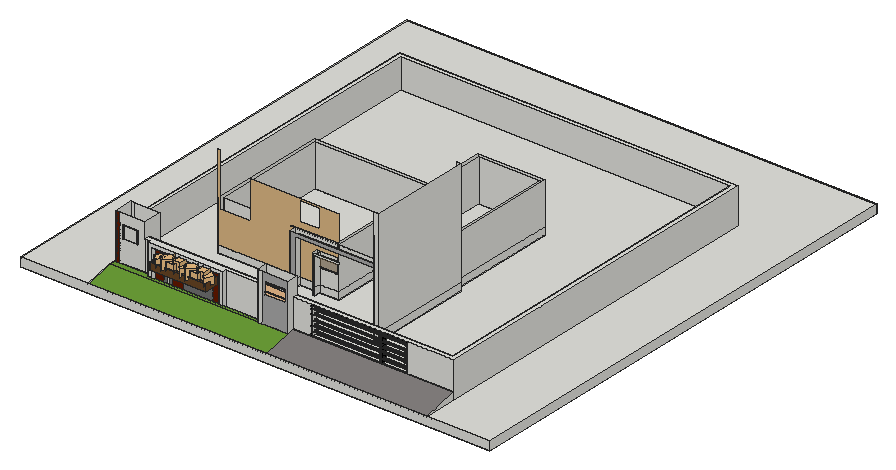
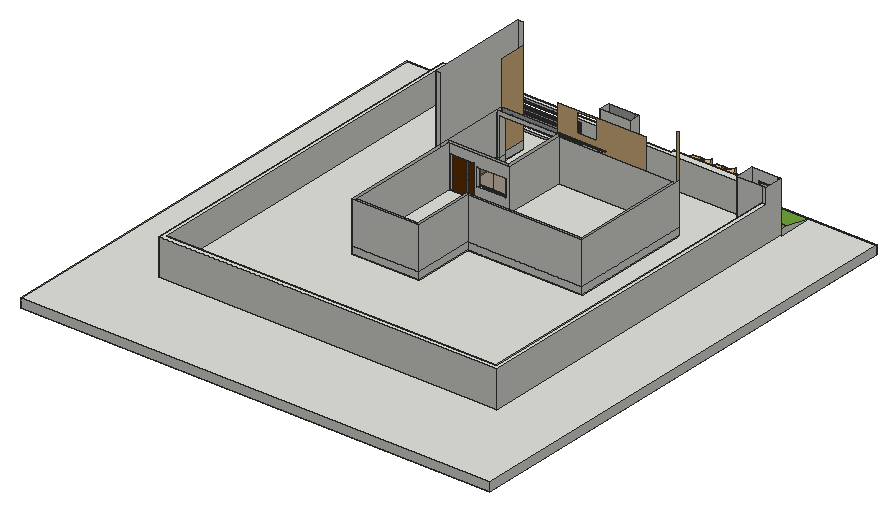
# SketchUp Ruby script. Lengths in millimetres.
U = 1.mm
M = Sketchup.active_model
def pt(a) = Geom::Point3d.new(a.map { |v| v * U })
def face(e, loops, mat)
  f = e.add_face(loops[0].map { |a| pt(a) })
  loops[1..].each { |l| e.add_face(l.map { |a| pt(a) }).erase! }
  f.material = f.back_material = mat if mat
  f
end
# faces: each face lists its corners as indices into pts; further lists are holes
def faces(e, pts, list, mat = nil) = list.each { |f| face(e, (f[0].is_a?(Array) ? f : [f]).map { |l| l.map { |i| pts[i] } }, mat) }
# xy, xz, yz: faces in a plane at the given z, y or x. An outline is a flat list of corners, or four numbers for a rectangle; further outlines are holes
def ring(l) = l.size == 4 ? [[l[0], l[1]], [l[2], l[1]], [l[2], l[3]], [l[0], l[3]]] : l.each_slice(2).to_a
def flat(e, list, mat, &to3) = list.each { |f| face(e, (f[0].is_a?(Array) ? f : [f]).map { |l| ring(l).map { |u, v| to3.(u, v) } }, mat) }
def xy(e, z, list, mat = nil) = flat(e, list, mat) { |x, y| [x, y, z] }
def xz(e, y, list, mat = nil) = flat(e, list, mat) { |x, z| [x, y, z] }
def yz(e, x, list, mat = nil) = flat(e, list, mat) { |y, z| [x, y, z] }
def lines(e, pts, list) = list.each { |a, b| e.add_line(pt(pts[a]), pt(pts[b])) }
# prism: a flat outline (further loops are holes) pulled along v
def prism(e, loops, v, mat = nil)
  f = face(e, loops, mat); d = Geom::Vector3d.new(v.map { |x| x * U })
  f.pushpull(f.normal.samedirection?(d) ? d.length : -d.length)
end
def box(e, o, s, mat = nil) = prism(e, [[o, [o[0] + s[0], o[1], o[2]], [o[0] + s[0], o[1] + s[1], o[2]], [o[0], o[1] + s[1], o[2]]]], [0, 0, s[2]], mat)
def at(x, y, z, deg = 0) = Geom::Transformation.translation(pt([x, y, z])) * Geom::Transformation.rotation(ORIGIN, Z_AXIS, deg.degrees)
def axes(o, x, y, z) = Geom::Transformation.new([*x, 0, *y, 0, *z, 0, *pt(o).to_a, 1])
def part(name) = M.definitions.add(name)
# library, detail: a bought-in or finely detailed component or shape, given as its bounding box
def library(name, o, s) = part(name).tap { |d| box(d.entities, o, s) }
def detail(e, o, s) = box(e.add_group.entities, o, s)
def put(e, d, t, mat = nil) = e.add_instance(d, t).tap { |i| i.material = mat if mat }
def group(e, t, mat = nil) = e.add_group.tap { |g| g.transformation = t; g.material = mat if mat }.entities
root = M.entities
M.materials.add("Material__1").color = [95, 70, 46]
M.materials.add("[Color B08]").color = [102, 25, 0]
M.materials.add("[Color C02]").color = [255, 204, 153]
M.materials.add("[Color C06]").color = [204, 102, 0]
M.materials.add("[Color C08]").color = [102, 51, 0]
M.materials.add("[Color M03]").color = [170, 170, 170]
M.materials.add("[Color M05]").color = [114, 114, 114]
M.materials.add("[Color M09]").color = [0, 0, 0]
M.materials.add("[Fencing Wood Old]").color = [132, 128, 126]
M.materials.add("[Grass Dark Green]").color = [106, 157, 55]
M.materials.add("[Translucent Glass Gray]").color = [128, 100, 65]
M.materials["[Translucent Glass Gray]"].alpha = 0.5
M.materials.add("[Wallpaper Stripe]1").color = [222, 185, 133]
M.materials.add("[Wood Veneer 01]").color = [104, 70, 37]
c1 = library("Areca palm plant",[0,0,0],[1247.1,929.7,1383.3])
c2 = library("Group20\#1",[-528.7,-433.9,96.3],[1012.6,1001.6,952.6])
c3 = library("Group\#130",[-186.5,-30.4,0],[982.4,909.6,1245.7])
c4 = library("Group38\#2",[355.8,722.5,-595.2],[471.9,465.1,987.8])
c5 = library("Group\#18",[-2151.2,-2287.7,-9.3],[4483.3,4448.3,4353.7])
c6 = library("Group\#74",[-2151.2,-2287.7,-9.3],[4483.3,4448.3,4353.7])
c7 = library("Group20\#2",[-528.7,-433.9,96.3],[1012.6,1001.6,952.6])
xy(root,-1719.3,[[[0,0,37484,38608],[24317.2,4921.6,24679,4921.6,24679,13178.8,24317.2,13178.8,24317.2,21945.9,18983.2,21945.9,18983.2,17069.1,9839.2,17069.1,9839.2,7467.9,15925.7,7467.9,15925.7,7006,16385.5,7006,16385.5,7467.9,17737,7467.9,17737,7006,17916.4,7006,17916.4,7467.9,19440.4,7467.9,19440.4,12344.7,24317.2,12344.7,24317.2,7467.9,24068.1,7467.9,24068.1,7006,24317.2,7006]]])
xy(root,-1062,[[0,0,5401.7,0,5401.7,2705.1,5428.7,2705.1,5428.7,31078.5,32435.2,31078.5,32435.2,0,37484,0,37484,38608,0,38608],[5401.7,0,32435.2,0,32435.2,2705.1,18869,2705.1,18869,2189.2,17189.8,2189.2,17189.8,2457.5,8186.8,2457.5,8186.8,2705.1,5401.7,2705.1],[8573.9,2457.5,13875.2,2705.1],[14222.2,2457.5,17189.8,2705.1]])
xy(root,-597.6,[[5401.7,2189.2,17189.8,2189.2,17189.8,2457.5,8186.8,2457.5,8186.8,2705.1,5401.7,2705.1]],"[Grass Dark Green]")
xy(root,-582.6,[[[7761.5,3056,32084.3,3056,32084.3,30727.6,5779.6,30727.6,5779.6,4232.4,7761.5,4232.4],[24317.2,4921.6,24317.2,7006,24068.1,7006,24068.1,7467.9,24317.2,7467.9,24317.2,12344.7,19440.4,12344.7,19440.4,7467.9,17916.4,7467.9,17916.4,7006,17737,7006,17737,7467.9,16385.5,7467.9,16385.5,7006,15925.7,7006,15925.7,7467.9,9839.2,7467.9,9839.2,17069.1,18983.2,17069.1,18983.2,21945.9,24317.2,21945.9,24317.2,13178.8,24679,13178.8,24679,4921.6]]])
xy(root,-453.1,[[21185.9,2705.1,26553.4,3056],[26740.8,2705.1,28682.4,3056]])
xy(root,-60,[[26604.3,2675,26678.9,2705.1]])
xy(root,0,[[24317.2,4921.6,24679,13178.8],[15925.7,7006,16385.5,7006,16385.5,7467.9,19440.4,7467.9,19440.4,12344.7,22064.1,12344.7,22064.1,12573.3,19211.8,12573.3,19211.8,7696.5,10067.8,7696.5,10067.8,16840.5,19211.8,16840.5,19211.8,21717.3,24088.6,21717.3,24088.6,12573.3,23941.7,12573.3,23941.7,12344.7,24317.2,12344.7,24317.2,21945.9,18983.2,21945.9,18983.2,17069.1,9839.2,17069.1,9839.2,7467.9,15925.7,7467.9],[17737,7006,17916.4,7467.9],[24068.1,7006,24317.2,7467.9],[10067.8,7696.5,19211.8,7696.5,19211.8,12573.3,24088.6,12573.3,24088.6,21717.3,19211.8,21717.3,19211.8,16840.5,10067.8,16840.5],
  [22064.1,12344.7,22164,12344.7,22164,12522.5,23841.8,12522.5,23841.8,12344.7,23941.7,12344.7,23941.7,12573.3,22064.1,12573.3],[22164,12344.7,23841.8,12522.5]])
xy(root,143.2,[[26604.3,2675,26678.9,2705.1]])
xy(root,489.4,[[9066,1643.1,13519,2705.1]])
xy(root,651.3,[[9192.3,1769.3,13392.7,2705.1]])
xy(root,971.6,[[19543.5,12344.7,21847.6,12573.3]])
xy(root,1081.4,[[23379.6,12446.3,23760.6,12522.5]])
xy(root,1091,[[9066,1643.1,13519,1643.1,13519,2705.1,13392.7,2705.1,13392.7,1769.3,9192.3,1769.3,9192.3,2705.1,9066,2705.1]],"[Wood Veneer 01]")
xy(root,1157.6,[[23379.6,12446.3,23760.6,12522.5]])
xy(root,1161.7,[[6020.4,2705.1,7206.3,2730.5]])
xy(root,1237.5,[[6096.2,2705.1,7130.5,2730.5]])
xy(root,1413.2,[[26604.3,2675,26678.9,2705.1]])
xy(root,1565.9,[[8573.9,2457.5,13875.2,2705.1]])
xy(root,1610.1,[[26604.3,2675,26678.9,2705.1]],"[Color M03]")
xy(root,1691.4,[[21185.9,2705.1,26553.4,3056],[26740.8,2705.1,28682.4,3056]])
xy(root,1820.9,[[8186.8,2457.5,14222.2,2457.5,14222.2,2705.1,17189.8,2705.1,17189.8,3052.8,19635.7,3052.8,19635.7,2705.1,32435.2,2705.1,32435.2,31078.5,5428.7,31078.5,5428.7,4232.4,5779.6,4232.4,5779.6,30727.6,32084.3,30727.6,32084.3,3056,7761.5,3056,7761.5,2705.1,8186.8,2705.1]])
xz(root,0,[[0,-1719.3,37484,-1062]])
xz(root,1643.1,[[9066,489.4,13519,1091]],"[Wood Veneer 01]")
xz(root,1769.3,[[9192.3,651.3,13392.7,1091]])
xz(root,2189.2,[[17189.8,-1062,17330.6,-597.6],[17330.6,-1062,17575.1,-597.6],[17575.1,-1062,18869,-597.6],[17330.6,-597.6,17575.1,3141.7]])
xz(root,2189.2,[[17767.7,1526.9,19436.2,1764.4],[17767.7,1764.4,19436.2,1796.7],[17767.7,1796.7,19436.2,2287.5]],"[Color C02]")
xz(root,2189.2,[[17189.8,-597.6,17330.6,3141.7],[[17575.1,-597.6,19635.7,3141.7],[17767.7,1526.9,19436.2,2536.5]]],"[Color M03]")
xz(root,2457.5,[[8186.8,-1062,8573.9,-597.6],[8573.9,-1062,13875.2,-597.6],[13875.2,-1062,14222.2,-597.6],[14222.2,-1062,17189.8,-597.6],[8186.8,-597.6,8573.9,-597.6,8573.9,1565.9,13875.2,1565.9,13875.2,-597.6,14222.2,-597.6,14222.2,1820.9,8186.8,1820.9]])
xz(root,2675,[[26604.3,-60,26678.9,143.2],[26604.3,1413.2,26678.9,1610.1]],"[Color M03]")
xz(root,2705.1,[[5401.7,-1062,5428.7,-597.6],[5428.7,-1062,5561.2,-597.6],[5561.2,-1062,5760.5,-597.6],[5760.5,-1062,7761.5,-597.6],[7761.5,-1062,8186.8,-597.6],
  [9523.8,-1062,9761.8,489.4],[14222.2,-1062,17189.8,1820.9],[18869,-1062,21056.4,-488.2],[21056.4,-1062,28811.9,-488.2],[28811.9,-1062,32435.2,-488.2],
  [5428.7,-597.6,5561.2,2994],[[5760.5,-597.6,7761.5,2994],[6020.4,1161.7,7206.3,2222.2]],[7761.5,-597.6,8186.8,1820.9],[19635.7,-488.2,21056.4,1820.9],[28811.9,-488.2,32435.2,1820.9],
  [26604.3,-60,26678.9,143.2],[9523.8,651.3,9761.8,1565.9],[6096.2,1237.5,7130.5,2146.4]])
xz(root,2705.1,[[8573.9,-1062,9295.9,-1062,9295.9,489.4,9066,489.4,9066,1091,9192.3,1091,9192.3,651.3,9295.9,651.3,9295.9,1565.9,8573.9,1565.9],[9989.6,-1062,10808,489.4],[13214.2,-1062,13875.2,-1062,13875.2,1565.9,13214.2,1565.9,13214.2,651.3,13392.7,651.3,13392.7,1091,13519,1091,13519,489.4,13214.2,489.4],[5561.2,-597.6,5760.5,2994],[9989.6,651.3,10808,1565.9]],"[Color B08]")
xz(root,2705.1,[[9295.9,-1062,9523.8,489.4],[9761.8,-1062,9989.6,489.4],[10808,-1062,13214.2,489.4],[9295.9,651.3,9523.8,1565.9],[9761.8,651.3,9989.6,1565.9],
  [10808,651.3,13214.2,1565.9]],"[Color M05]")
xz(root,2705.1,[[[21056.4,-488.2,28811.9,1820.9],[21185.9,-453.1,28682.4,1691.4]],[[26553.4,-453.1,26740.8,1691.4],[26604.3,-60,26678.9,143.2],[26604.3,1413.2,26678.9,1610.1]]],"[Color M09]")
xz(root,2730.5,[[[6020.4,1161.7,7206.3,2222.2],[6096.2,1237.5,7130.5,2146.4]]])
xz(root,3052.8,[[17189.8,1820.9,19635.7,3141.7]])
xz(root,3056,[[[7761.5,-582.6,32084.3,1820.9],[21185.9,-453.1,26553.4,1691.4],[26740.8,-453.1,28682.4,1691.4]]])
xz(root,4232.4,[[5779.6,-582.6,7761.5,2994],[5428.7,1820.9,5779.6,2994]])
xz(root,4921.6,[[24317.2,-1719.3,24679,-582.6],[24317.2,-582.6,24679,0],[24317.2,0,24679,8532.8]])
xz(root,7006,[[15925.7,-1719.3,16385.5,-582.6],[17737,-1719.3,17916.4,-582.6],[24068.1,-1719.3,24317.2,-582.6],[15925.7,-582.6,16385.5,0],[17737,-582.6,17916.4,0],
  [24068.1,-582.6,24317.2,0],[17737,0,17916.4,0,17916.4,2265.6,19853.2,2265.6,19853.2,2420.1,17737,2420.1]])
xz(root,7006,[[15925.7,0,16385.5,0,16385.5,3053.2,24068.1,3053.2,24068.1,0,24317.2,0,24317.2,3352.8,15925.7,3352.8]],"[Color M03]")
xz(root,7467.9,[[9839.2,-1719.3,15925.7,-582.6],[16385.5,-1719.3,17737,-582.6],[17916.4,-1719.3,19440.4,-582.6],[24068.1,-1719.3,24317.2,-582.6],[9839.2,-582.6,15925.7,0],
  [16385.5,-582.6,17737,0],[17916.4,-582.6,19440.4,0],[24068.1,-582.6,24317.2,0],[17737,0,17916.4,2265.6],[17916.4,0,19440.4,1219.2],
  [24068.1,0,24068.1,3053.2,19440.4,3053.2,19440.4,3352.8,24317.2,3352.8,24317.2,0]])
xz(root,7467.9,[[[17916.4,1219.2,19440.4,2133.6],[17964.1,1266.9,19392.7,2085.9]]],"[Color B08]")
xz(root,7467.9,[[17964.1,1266.9,19392.7,2085.9]],"[Translucent Glass Gray]")
xz(root,7467.9,[[[9839.2,0,15925.7,0,15925.7,3352.8,23273.7,3352.8,23273.7,3388.1,15532.7,3388.1,15532.7,3920.5,15634.5,3920.5,15634.5,3497.3,19430.1,3497.3,19430.1,5591.3,12413.6,5591.3,12413.6,2590.3,9937.1,2590.3,9937.1,6850.1,9839.2,6850.1],[16385.5,3962.4,17916.4,5486.4]],[16385.5,0,17737,0,17737,2420.1,19440.4,2420.1,19440.4,3053.2,16385.5,3053.2]],"[Wallpaper Stripe]1")
xz(root,7696.5,[[10067.8,0,19211.8,3352.8]])
xz(root,12344.7,[[19440.4,-1719.3,24317.2,-582.6],[19440.4,-582.6,24317.2,0],[[19440.4,0,22064.1,0,22064.1,2627.4,23941.7,2627.4,23941.7,0,24317.2,0,24317.2,3352.8,19440.4,3352.8],[19543.5,971.6,21847.6,2395.6]]])
xz(root,12344.7,[[22064.1,0,22164,0,22164,2527.5,23841.8,2527.5,23841.8,0,23941.7,0,23941.7,2627.4,22064.1,2627.4]],"[Color C08]")
xz(root,12344.7,[[[19543.5,971.6,21847.6,2395.6],[19613.2,1041.2,21777.9,2325.9]]],"[Color M09]")
xz(root,12344.7,[[19613.2,1041.2,20695.5,2325.9],[20695.5,1041.2,21777.9,2325.9]],"[Translucent Glass Gray]")
xz(root,12446.3,[[23379.6,1081.4,23760.6,1157.6]])
xz(root,12522.5,[[22528.5,0,22698.2,2527.5]],"[Color C06]")
xz(root,12522.5,[[22164,0,22528.5,2527.5],[[22698.2,0,23841.8,2527.5],[23379.6,1081.4,23760.6,1157.6]]],"[Color C08]")
xz(root,12573.3,[[[19211.8,0,19211.8,3352.8,24088.6,3352.8,24088.6,0,23941.7,0,23941.7,2627.4,22064.1,2627.4,22064.1,0],[19543.5,971.6,21847.6,2395.6]]])
xz(root,13178.8,[[24317.2,-1719.3,24679,-582.6],[24317.2,-582.6,24679,0],[24317.2,0,24679,8532.8]])
xz(root,16840.5,[[10067.8,0,19211.8,3352.8]])
xz(root,17069.1,[[9839.2,-1719.3,18983.2,-582.6],[9839.2,-582.6,18983.2,0],[9839.2,0,18983.2,3352.8]])
xz(root,21717.3,[[19211.8,0,24088.6,3352.8]])
xz(root,21945.9,[[18983.2,-1719.3,24317.2,-582.6],[18983.2,-582.6,24317.2,0],[18983.2,0,24317.2,3352.8]])
xz(root,30727.6,[[5779.6,-582.6,32084.3,1820.9]])
xz(root,31078.5,[[5428.7,-1062,32435.2,1820.9]])
xz(root,38608,[[0,-1719.3,37484,-1062]])
yz(root,0,[[0,-1719.3,38608,-1062]])
yz(root,5401.7,[[0,-1062,2189.2,-597.6,2705.1,-597.6,2705.1,-1062]])
yz(root,5428.7,[[2705.1,-1062,2705.1,2994,4232.4,2994,4232.4,1820.9,31078.5,1820.9,31078.5,-1062]])
yz(root,5779.6,[[4232.4,-582.6,30727.6,1820.9]])
yz(root,6020.4,[[2705.1,1161.7,2730.5,2222.2]])
yz(root,6096.2,[[2705.1,1237.5,2730.5,2146.4]])
yz(root,7130.5,[[2705.1,1237.5,2730.5,2146.4]])
yz(root,7206.3,[[2705.1,1161.7,2730.5,2222.2]])
yz(root,7761.5,[[[3056,-582.6,4232.4,-582.6,4232.4,2994,2705.1,2994,2705.1,1820.9,3056,1820.9],[2877.4,2559.6,2857.6,2562.2,2839.3,2569.8,2823.5,2581.9,2811.4,2597.7,2803.7,2616.1,2801.2,2635.8,2803.7,2655.5,2811.4,2673.9,2823.5,2689.7,2839.3,2701.8,2857.6,2709.4,2877.4,2712,2897.1,2709.4,2915.5,2701.8,2931.2,2689.7,2943.3,2673.9,2951,2655.5,2953.6,2635.8,2951,2616.1,2943.3,2597.7,2931.2,2581.9,2915.5,2569.8,2897.1,2562.2],[2877.4,1870.6,2857.6,1873.2,2839.3,1880.8,2823.5,1892.9,2811.4,1908.7,2803.7,1927.1,2801.2,1946.8,2803.7,1966.5,2811.4,1984.9,2823.5,2000.7,2839.3,2012.8,2857.6,2020.4,2877.4,2023,2897.1,2020.4,2915.5,2012.8,2931.2,2000.7,2943.3,1984.9,2951,1966.5,2953.6,1946.8,2951,1927.1,2943.3,1908.7,2931.2,1892.9,2915.5,1880.8,2897.1,1873.2],[2877.4,2234.1,2857.6,2236.7,2839.3,2244.3,2823.5,2256.5,2811.4,2272.2,2803.7,2290.6,2801.2,2310.3,2803.7,2330.1,2811.4,2348.4,2823.5,2364.2,2839.3,2376.3,2857.6,2383.9,2877.4,2386.5,2897.1,2383.9,2915.5,2376.3,2931.2,2364.2,2943.3,2348.4,2951,2330.1,2953.6,2310.3,2951,2290.6,2943.3,2272.2,2931.2,2256.5,2915.5,2244.3,2897.1,2236.7]]])
yz(root,8186.8,[[2457.5,-1062,2705.1,-712.8],[2457.5,-712.8,2705.1,-597.6],[2457.5,-597.6,2705.1,1820.9]])
yz(root,8573.9,[[2457.5,-1062,2705.1,1565.9]])
yz(root,9066,[[1643.1,489.4,2705.1,1091]],"[Wood Veneer 01]")
yz(root,9192.3,[[1769.3,651.3,2705.1,1091]])
yz(root,9839.2,[[7467.9,-1719.3,17069.1,-582.6],[7467.9,-582.6,17069.1,0],[7467.9,0,17069.1,3352.8]])
yz(root,10067.8,[[7696.5,0,16840.5,3352.8]])
yz(root,13392.7,[[1769.3,651.3,2705.1,1091]])
yz(root,13519,[[1643.1,489.4,2705.1,1091]],"[Wood Veneer 01]")
yz(root,13875.2,[[2457.5,-1062,2705.1,1565.9]])
yz(root,14222.2,[[2457.5,-1062,2705.1,1820.9]])
yz(root,15925.7,[[7006,-1719.3,7467.9,-582.6],[7006,-582.6,7467.9,0],[7006,0,7467.9,3352.8]])
yz(root,16385.5,[[7006,-1719.3,7467.9,-582.6],[7006,-582.6,7467.9,0],[7006,0,7467.9,3053.2]])
yz(root,17189.8,[[2189.2,-1062,2457.5,-597.6],[[2457.5,-1062,2457.5,-597.6,2189.2,-597.6,2189.2,3141.7,3052.8,3141.7,3052.8,1820.9,2705.1,1820.9,2705.1,-1062],[2877.4,1870.6,2897.1,1873.2,2915.5,1880.8,2931.2,1892.9,2943.3,1908.7,2951,1927.1,2953.6,1946.8,2951,1966.5,2943.3,1984.9,2931.2,2000.7,2915.5,2012.8,2897.1,2020.4,2877.4,2023,2857.6,2020.4,2839.3,2012.8,2823.5,2000.7,2811.4,1984.9,2803.7,1966.5,2801.2,1946.8,2803.7,1927.1,2811.4,1908.7,2823.5,1892.9,2839.3,1880.8,2857.6,1873.2]]])
yz(root,17737,[[7006,-1719.3,7467.9,-582.6],[7006,-582.6,7467.9,0],[7006,0,7467.9,2420.1]])
yz(root,17916.4,[[7006,-1719.3,7467.9,-582.6],[7006,-582.6,7467.9,0],[7006,0,7467.9,2265.6]])
yz(root,18869,[[2189.2,-1062,2189.2,-597.6,2705.1,-488.2,2705.1,-1062]])
yz(root,18983.2,[[17069.1,-1719.3,21945.9,-582.6],[17069.1,-582.6,21945.9,0],[17069.1,0,21945.9,3352.8]])
yz(root,19211.8,[[7696.5,0,12573.3,3352.8],[16840.5,0,21717.3,3352.8]])
yz(root,19440.4,[[7467.9,-1719.3,12344.7,-582.6],[7467.9,-582.6,12344.7,0],[7467.9,0,12344.7,3352.8]])
yz(root,19543.5,[[12344.7,971.6,12573.3,2395.6]])
yz(root,19635.7,[[2189.2,-597.6,2705.1,-488.2,2705.1,1820.9,3052.8,1820.9,3052.8,3141.7,2189.2,3141.7]])
yz(root,21185.9,[[[2705.1,-453.1,3056,1691.4],[2868.1,574.9,2848.4,577.5,2830,585.1,2814.3,597.2,2802.2,613,2794.5,631.4,2791.9,651.1,2794.5,670.8,2802.2,689.2,2814.3,705,2830,717.1,2848.4,724.7,2868.1,727.3,2887.9,724.7,2906.2,717.1,2922,705,2934.1,689.2,2941.7,670.8,2944.3,651.1,2941.7,631.4,2934.1,613,2922,597.2,2906.2,585.1,2887.9,577.5],[2868.1,982.9,2848.4,985.5,2830,993.1,2814.3,1005.2,2802.2,1021,2794.5,1039.4,2791.9,1059.1,2794.5,1078.8,2802.2,1097.2,2814.3,1113,2830,1125.1,2848.4,1132.7,2868.1,1135.3,2887.9,1132.7,2906.2,1125.1,2922,1113,2934.1,1097.2,2941.7,1078.8,2944.3,1059.1,2941.7,1039.4,2934.1,1021,2922,1005.2,2906.2,993.1,2887.9,985.5],[2868.1,166.9,2848.4,169.5,2830,177.1,2814.3,189.2,2802.2,205,2794.5,223.4,2791.9,243.1,2794.5,262.8,2802.2,281.2,2814.3,297,2830,309.1,2848.4,316.7,2868.1,319.3,2887.9,316.7,2906.2,309.1,2922,297,2934.1,281.2,2941.7,262.8,2944.3,243.1,2941.7,223.4,2934.1,205,2922,189.2,2906.2,177.1,2887.9,169.5],[2868.1,-241.1,2848.4,-238.5,2830,-230.9,2814.3,-218.7,2802.2,-203,2794.5,-184.6,2791.9,-164.9,2794.5,-145.1,2802.2,-126.8,2814.3,-111,2830,-98.9,2848.4,-91.3,2868.1,-88.7,2887.9,-91.3,2906.2,-98.9,2922,-111,2934.1,-126.8,2941.7,-145.1,2944.3,-164.9,2941.7,-184.6,2934.1,-203,2922,-218.7,2906.2,-230.9,2887.9,-238.5],[2868.1,1390.9,2848.4,1393.5,2830,1401.1,2814.3,1413.2,2802.2,1429,2794.5,1447.4,2791.9,1467.1,2794.5,1486.8,2802.2,1505.2,2814.3,1521,2830,1533.1,2848.4,1540.7,2868.1,1543.3,2887.9,1540.7,2906.2,1533.1,2922,1521,2934.1,1505.2,2941.7,1486.8,2944.3,1467.1,2941.7,1447.4,2934.1,1429,2922,1413.2,2906.2,1401.1,2887.9,1393.5]]])
yz(root,21847.6,[[12344.7,971.6,12573.3,2395.6]])
yz(root,22064.1,[[12344.7,0,12573.3,2627.4]])
yz(root,22164,[[12344.7,0,12522.5,2527.5]],"[Color C08]")
yz(root,23379.6,[[12446.3,1081.4,12522.5,1157.6]])
yz(root,23760.6,[[12446.3,1081.4,12522.5,1157.6]])
yz(root,23841.8,[[12344.7,0,12522.5,2527.5]],"[Color C08]")
yz(root,23941.7,[[12344.7,0,12573.3,2627.4]])
yz(root,24068.1,[[7006,-1719.3,7467.9,-582.6],[7006,-582.6,7467.9,0],[7006,0,7467.9,3053.2]])
yz(root,24088.6,[[12573.3,0,21717.3,3352.8]])
yz(root,24317.2,[[4921.6,-1719.3,7006,-582.6],[7467.9,-1719.3,12344.7,-582.6],[13178.8,-1719.3,21945.9,-582.6],[4921.6,-582.6,7006,0],[7467.9,-582.6,12344.7,0],
  [13178.8,-582.6,21945.9,0],[7006,0,7467.9,3352.8],[7467.9,0,12344.7,3352.8],[12344.7,0,13178.8,3352.8],[13178.8,0,21945.9,3352.8]])
yz(root,24317.2,[[4921.6,0,7006,6850.1]],"[Wallpaper Stripe]1")
yz(root,24679,[[4921.6,-1719.3,13178.8,-582.6],[4921.6,-582.6,13178.8,0],[4921.6,0,13178.8,8532.8]])
yz(root,26553.4,[[2705.1,-453.1,3056,1691.4]],"[Color M09]")
yz(root,26604.3,[[2675,-60,2705.1,143.2],[2675,1413.2,2705.1,1610.1]],"[Color M03]")
yz(root,26678.9,[[2675,-60,2705.1,143.2]])
yz(root,26678.9,[[2675,1413.2,2705.1,1610.1]],"[Color M03]")
yz(root,26740.8,[[2705.1,-453.1,3056,1691.4]],"[Color M09]")
yz(root,28663,[[2868.1,166.9,2887.9,169.5,2906.2,177.1,2922,189.2,2934.1,205,2941.7,223.4,2944.3,243.1,2941.7,262.8,2934.1,281.2,2922,297,2906.2,309.1,2887.9,316.7,2868.1,319.3,2848.4,316.7,2830,309.1,2814.3,297,2802.2,281.2,2794.5,262.8,2791.9,243.1,2794.5,223.4,2802.2,205,2814.3,189.2,2830,177.1,2848.4,169.5]])
yz(root,28664.6,[[2868.1,-241.1,2887.9,-238.5,2906.2,-230.9,2922,-218.7,2934.1,-203,2941.7,-184.6,2944.3,-164.9,2941.7,-145.1,2934.1,-126.8,2922,-111,2906.2,-98.9,2887.9,-91.3,2868.1,-88.7,2848.4,-91.3,2830,-98.9,2814.3,-111,2802.2,-126.8,2794.5,-145.1,2791.9,-164.9,2794.5,-184.6,2802.2,-203,2814.3,-218.7,2830,-230.9,2848.4,-238.5]])
yz(root,28666.2,[[2868.1,574.9,2887.9,577.5,2906.2,585.1,2922,597.2,2934.1,613,2941.7,631.4,2944.3,651.1,2941.7,670.8,2934.1,689.2,2922,705,2906.2,717.1,2887.9,724.7,2868.1,727.3,2848.4,724.7,2830,717.1,2814.3,705,2802.2,689.2,2794.5,670.8,2791.9,651.1,2794.5,631.4,2802.2,613,2814.3,597.2,2830,585.1,2848.4,577.5]])
yz(root,28682.4,[[[2705.1,-453.1,3056,1691.4],[2868.1,982.9,2887.9,985.5,2906.2,993.1,2922,1005.2,2934.1,1021,2941.7,1039.4,2944.3,1059.1,2941.7,1078.8,2934.1,1097.2,2922,1113,2906.2,1125.1,2887.9,1132.7,2868.1,1135.3,2848.4,1132.7,2830,1125.1,2814.3,1113,2802.2,1097.2,2794.5,1078.8,2791.9,1059.1,2794.5,1039.4,2802.2,1021,2814.3,1005.2,2830,993.1,2848.4,985.5],[2868.1,1390.9,2887.9,1393.5,2906.2,1401.1,2922,1413.2,2934.1,1429,2941.7,1447.4,2944.3,1467.1,2941.7,1486.8,2934.1,1505.2,2922,1521,2906.2,1533.1,2887.9,1540.7,2868.1,1543.3,2848.4,1540.7,2830,1533.1,2814.3,1521,2802.2,1505.2,2794.5,1486.8,2791.9,1467.1,2794.5,1447.4,2802.2,1429,2814.3,1413.2,2830,1401.1,2848.4,1393.5]]])
yz(root,32084.3,[[3056,-582.6,30727.6,1820.9]])
yz(root,32435.2,[[0,-1062,2705.1,-1062,2705.1,-488.2],[2705.1,-1062,31078.5,1820.9]])
yz(root,37484,[[0,-1719.3,38608,-1062]])
p = [[5401.7,0,-1062],[19635.7,0,-1062],[19635.7,2189.2,-597.6],[18869,2189.2,-597.6],[17575.1,2189.2,-597.6],[17330.6,2189.2,-597.6],
  [17189.8,2189.2,-597.6],[5401.7,2189.2,-597.6],[19635.7,2705.1,-488.2],[32435.2,0,-1062],[32435.2,2705.1,-488.2],[28811.9,2705.1,-488.2],
  [21056.4,2705.1,-488.2],[18869,2705.1,-488.2],[21185.9,2848.4,-238.5],[21185.9,2868.1,-241.1],[28664.6,2868.1,-241.1],[28664.6,2848.4,-238.5],
  [21185.9,2887.9,-238.5],[28664.6,2887.9,-238.5],[21185.9,2830,-230.9],[28664.6,2830,-230.9],[21185.9,2906.2,-230.9],[28664.6,2906.2,-230.9],
  [21185.9,2814.3,-218.7],[28664.6,2814.3,-218.7],[21185.9,2922,-218.7],[28664.6,2922,-218.7],[21185.9,2802.2,-203],[28664.6,2802.2,-203],
  [21185.9,2934.1,-203],[28664.6,2934.1,-203],[21185.9,2794.5,-184.6],[28664.6,2794.5,-184.6],[21185.9,2941.7,-184.6],[28664.6,2941.7,-184.6],
  [21185.9,2791.9,-164.9],[28664.6,2791.9,-164.9],[21185.9,2944.3,-164.9],[28664.6,2944.3,-164.9],[21185.9,2794.5,-145.1],[28664.6,2794.5,-145.1],
  [21185.9,2941.7,-145.1],[28664.6,2941.7,-145.1],[21185.9,2802.2,-126.8],[28664.6,2802.2,-126.8],[21185.9,2934.1,-126.8],[28664.6,2934.1,-126.8],
  [21185.9,2814.3,-111],[28664.6,2814.3,-111],[21185.9,2922,-111],[28664.6,2922,-111],[21185.9,2830,-98.9],[28664.6,2830,-98.9],
  [21185.9,2906.2,-98.9],[28664.6,2906.2,-98.9],[21185.9,2848.4,-91.3],[28664.6,2848.4,-91.3],[21185.9,2887.9,-91.3],[28664.6,2887.9,-91.3],
  [21185.9,2868.1,-88.7],[28664.6,2868.1,-88.7],[22274.5,12522.5,2527.5],[22274.5,12344.7,0],[22454.8,12344.7,0],[22454.8,12522.5,2527.5],
  [21185.9,2848.4,169.5],[21185.9,2868.1,166.9],[28663,2868.1,166.9],[28663,2848.4,169.5],[21185.9,2887.9,169.5],[28663,2887.9,169.5],
  [21185.9,2830,177.1],[28663,2830,177.1],[21185.9,2906.2,177.1],[28663,2906.2,177.1],[21185.9,2814.3,189.2],[28663,2814.3,189.2],
  [21185.9,2922,189.2],[28663,2922,189.2],[21185.9,2802.2,205],[28663,2802.2,205],[21185.9,2934.1,205],[28663,2934.1,205],
  [21185.9,2794.5,223.4],[28663,2794.5,223.4],[21185.9,2941.7,223.4],[28663,2941.7,223.4],[21185.9,2791.9,243.1],[28663,2791.9,243.1],
  [21185.9,2944.3,243.1],[28663,2944.3,243.1],[21185.9,2794.5,262.8],[28663,2794.5,262.8],[21185.9,2941.7,262.8],[28663,2941.7,262.8],
  [21185.9,2802.2,281.2],[28663,2802.2,281.2],[21185.9,2934.1,281.2],[28663,2934.1,281.2],[21185.9,2814.3,297],[28663,2814.3,297],
  [21185.9,2922,297],[28663,2922,297],[21185.9,2830,309.1],[28663,2830,309.1],[21185.9,2906.2,309.1],[28663,2906.2,309.1],
  [21185.9,2848.4,316.7],[28663,2848.4,316.7],[21185.9,2887.9,316.7],[28663,2887.9,316.7],[21185.9,2868.1,319.3],[28663,2868.1,319.3],
  [21185.9,2848.4,577.5],[21185.9,2868.1,574.9],[28666.2,2868.1,574.9],[28666.2,2848.4,577.5],[21185.9,2887.9,577.5],[28666.2,2887.9,577.5],
  [21185.9,2830,585.1],[28666.2,2830,585.1],[21185.9,2906.2,585.1],[28666.2,2906.2,585.1],[21185.9,2814.3,597.2],[28666.2,2814.3,597.2],
  [21185.9,2922,597.2],[28666.2,2922,597.2],[21185.9,2802.2,613],[28666.2,2802.2,613],[21185.9,2934.1,613],[28666.2,2934.1,613],
  [21185.9,2794.5,631.4],[28666.2,2794.5,631.4],[21185.9,2941.7,631.4],[28666.2,2941.7,631.4],[21185.9,2791.9,651.1],[28666.2,2791.9,651.1],
  [21185.9,2944.3,651.1],[28666.2,2944.3,651.1],[21185.9,2794.5,670.8],[28666.2,2794.5,670.8],[21185.9,2941.7,670.8],[28666.2,2941.7,670.8],
  [21185.9,2802.2,689.2],[28666.2,2802.2,689.2],[21185.9,2934.1,689.2],[28666.2,2934.1,689.2],[21185.9,2814.3,705],[28666.2,2814.3,705],
  [21185.9,2922,705],[28666.2,2922,705],[21185.9,2830,717.1],[28666.2,2830,717.1],[21185.9,2906.2,717.1],[28666.2,2906.2,717.1],
  [21185.9,2848.4,724.7],[28666.2,2848.4,724.7],[21185.9,2887.9,724.7],[28666.2,2887.9,724.7],[21185.9,2868.1,727.3],[28666.2,2868.1,727.3],
  [21185.9,2848.4,985.5],[21185.9,2868.1,982.9],[28682.4,2868.1,982.9],[28682.4,2848.4,985.5],[21185.9,2887.9,985.5],[28682.4,2887.9,985.5],
  [21185.9,2830,993.1],[28682.4,2830,993.1],[21185.9,2906.2,993.1],[28682.4,2906.2,993.1],[21185.9,2814.3,1005.2],[28682.4,2814.3,1005.2],
  [21185.9,2922,1005.2],[28682.4,2922,1005.2],[21185.9,2802.2,1021],[28682.4,2802.2,1021],[21185.9,2934.1,1021],[28682.4,2934.1,1021],
  [21185.9,2794.5,1039.4],[28682.4,2794.5,1039.4],[21185.9,2941.7,1039.4],[28682.4,2941.7,1039.4],[21185.9,2791.9,1059.1],[28682.4,2791.9,1059.1],
  [21185.9,2944.3,1059.1],[28682.4,2944.3,1059.1],[21185.9,2794.5,1078.8],[28682.4,2794.5,1078.8],[21185.9,2941.7,1078.8],[28682.4,2941.7,1078.8],
  [21185.9,2802.2,1097.2],[28682.4,2802.2,1097.2],[21185.9,2934.1,1097.2],[28682.4,2934.1,1097.2],[21185.9,2814.3,1113],[28682.4,2814.3,1113],
  [21185.9,2922,1113],[28682.4,2922,1113],[21185.9,2830,1125.1],[28682.4,2830,1125.1],[21185.9,2906.2,1125.1],[28682.4,2906.2,1125.1],
  [21185.9,2848.4,1132.7],[28682.4,2848.4,1132.7],[21185.9,2887.9,1132.7],[28682.4,2887.9,1132.7],[21185.9,2868.1,1135.3],[28682.4,2868.1,1135.3],
  [21185.9,2848.4,1393.5],[21185.9,2868.1,1390.9],[28682.4,2868.1,1390.9],[28682.4,2848.4,1393.5],[21185.9,2887.9,1393.5],[28682.4,2887.9,1393.5],
  [21185.9,2830,1401.1],[28682.4,2830,1401.1],[21185.9,2906.2,1401.1],[28682.4,2906.2,1401.1],[21185.9,2814.3,1413.2],[28682.4,2814.3,1413.2],
  [21185.9,2922,1413.2],[28682.4,2922,1413.2],[21185.9,2802.2,1429],[28682.4,2802.2,1429],[21185.9,2934.1,1429],[28682.4,2934.1,1429],
  [21185.9,2794.5,1447.4],[28682.4,2794.5,1447.4],[21185.9,2941.7,1447.4],[28682.4,2941.7,1447.4],[21185.9,2791.9,1467.1],[28682.4,2791.9,1467.1],
  [21185.9,2944.3,1467.1],[28682.4,2944.3,1467.1],[21185.9,2794.5,1486.8],[28682.4,2794.5,1486.8],[21185.9,2941.7,1486.8],[28682.4,2941.7,1486.8],
  [21185.9,2802.2,1505.2],[28682.4,2802.2,1505.2],[21185.9,2934.1,1505.2],[28682.4,2934.1,1505.2],[21185.9,2814.3,1521],[28682.4,2814.3,1521],
  [21185.9,2922,1521],[28682.4,2922,1521],[21185.9,2830,1533.1],[28682.4,2830,1533.1],[21185.9,2906.2,1533.1],[28682.4,2906.2,1533.1],
  [21185.9,2848.4,1540.7],[28682.4,2848.4,1540.7],[21185.9,2887.9,1540.7],[28682.4,2887.9,1540.7],[21185.9,2868.1,1543.3],[28682.4,2868.1,1543.3]]
faces(root,p,[[0,1,2,3,4,5,6,7]],"[Grass Dark Green]")
faces(root,p,[[8,2,1,9,10,11,12]],"[Fencing Wood Old]")
faces(root,p,[[13,3,2,8]])
faces(root,p,[[14,15,16,17],[15,18,19,16],[20,14,17,21],[18,22,23,19],[24,20,21,25],[22,26,27,23],[28,24,25,29],[26,30,31,27],
  [32,28,29,33],[30,34,35,31],[36,32,33,37],[34,38,39,35],[40,36,37,41],[38,42,43,39],[44,40,41,45],[42,46,47,43],
  [48,44,45,49],[46,50,51,47],[52,48,49,53],[50,54,55,51],[56,52,53,57],[54,58,59,55],[60,56,57,61],[58,60,61,59],
  [66,67,68,69],[67,70,71,68],[72,66,69,73],[70,74,75,71],[76,72,73,77],[74,78,79,75],[80,76,77,81],[78,82,83,79],
  [84,80,81,85],[82,86,87,83],[88,84,85,89],[86,90,91,87],[92,88,89,93],[90,94,95,91],[96,92,93,97],[94,98,99,95],
  [100,96,97,101],[98,102,103,99],[104,100,101,105],[102,106,107,103],[108,104,105,109],[106,110,111,107],[112,108,109,113],[110,112,113,111],
  [114,115,116,117],[115,118,119,116],[120,114,117,121],[118,122,123,119],[124,120,121,125],[122,126,127,123],[128,124,125,129],[126,130,131,127],
  [132,128,129,133],[130,134,135,131],[136,132,133,137],[134,138,139,135],[140,136,137,141],[138,142,143,139],[144,140,141,145],[142,146,147,143],
  [148,144,145,149],[146,150,151,147],[152,148,149,153],[150,154,155,151],[156,152,153,157],[154,158,159,155],[160,156,157,161],[158,160,161,159],
  [162,163,164,165],[163,166,167,164],[168,162,165,169],[166,170,171,167],[172,168,169,173],[170,174,175,171],[176,172,173,177],[174,178,179,175],
  [180,176,177,181],[178,182,183,179],[184,180,181,185],[182,186,187,183],[188,184,185,189],[186,190,191,187],[192,188,189,193],[190,194,195,191],
  [196,192,193,197],[194,198,199,195],[200,196,197,201],[198,202,203,199],[204,200,201,205],[202,206,207,203],[208,204,205,209],[206,208,209,207],
  [210,211,212,213],[211,214,215,212],[216,210,213,217],[214,218,219,215],[220,216,217,221],[218,222,223,219],[224,220,221,225],[222,226,227,223],
  [228,224,225,229],[226,230,231,227],[232,228,229,233],[230,234,235,231],[236,232,233,237],[234,238,239,235],[240,236,237,241],[238,242,243,239],
  [244,240,241,245],[242,246,247,243],[248,244,245,249],[246,250,251,247],[252,248,249,253],[250,254,255,251],[256,252,253,257],[254,256,257,255]],"[Color M09]")
faces(root,p,[[62,63,64,65]],"[Color C06]")
g1 = group(root,at(26544.9,2547.8,38.5),"[Color M03]")
xy(g1,1500.2,[[95.2,63.3,103.5,64.4,111.2,67.6,117.8,72.7,122.9,79.3,126.1,87,127.2,95.2,126.1,103.5,122.9,111.2,117.8,117.8,111.2,122.9,103.5,126.1,95.2,127.2,87,126.1,79.3,122.9,72.7,117.8,67.6,111.2,64.4,103.5,63.3,95.2,64.4,87,67.6,79.3,72.7,72.7,79.3,67.6,87,64.4]])
p = [[95.2,63.3,1500.2],[87,64.4,1500.2],[87,64.4,0],[95.2,63.3,0],[103.5,64.4,1500.2],[103.5,64.4,0],
  [79.3,67.6,1500.2],[79.3,67.6,0],[111.2,67.6,1500.2],[111.2,67.6,0],[72.7,72.7,1500.2],[72.7,72.7,0],
  [117.8,72.7,1500.2],[117.8,72.7,0],[67.6,79.3,1500.2],[67.6,79.3,0],[122.9,79.3,1500.2],[122.9,79.3,0],
  [64.4,87,1500.2],[64.4,87,0],[126.1,87,1500.2],[126.1,87,0],[63.3,95.2,1500.2],[63.3,95.2,0],
  [127.2,95.2,1500.2],[127.2,95.2,0],[64.4,103.5,1500.2],[64.4,103.5,0],[126.1,103.5,1500.2],[126.1,103.5,0],
  [67.6,111.2,1500.2],[67.6,111.2,0],[122.9,111.2,1500.2],[122.9,111.2,0],[72.7,117.8,1500.2],[72.7,117.8,0],
  [117.8,117.8,1500.2],[117.8,117.8,0],[79.3,122.9,1500.2],[79.3,122.9,0],[111.2,122.9,1500.2],[111.2,122.9,0],
  [87,126.1,1500.2],[87,126.1,0],[103.5,126.1,1500.2],[103.5,126.1,0],[95.2,127.2,1500.2],[95.2,127.2,0]]
faces(g1,p,[[0,1,2,3],[4,0,3,5],[1,6,7,2],[8,4,5,9],[6,10,11,7],[12,8,9,13],[10,14,15,11],[16,12,13,17],
  [14,18,19,15],[20,16,17,21],[18,22,23,19],[24,20,21,25],[22,26,27,23],[28,24,25,29],[26,30,31,27],[32,28,29,33],
  [30,34,35,31],[36,32,33,37],[34,38,39,35],[40,36,37,41],[38,42,43,39],[44,40,41,45],[42,46,47,43],[46,44,45,47]])
g2 = group(root,at(9158.1,2518.6,791.8))
xy(g2,19.9,[[61.6,-749.3,4234.6,-103.7]],"Material__1")
xz(g2,-749.3,[[61.6,19.9,4234.6,186.9]])
xz(g2,-103.7,[[61.6,19.9,4234.6,186.9]])
yz(g2,61.6,[[-749.3,19.9,-103.7,186.9]])
yz(g2,4234.6,[[-749.3,19.9,-103.7,186.9]])
put(g2,c1,axes([1019.4,224.3,0.7],[-0.41066,-0.47672,0],[0.38724,-0.70036,0],[0,0,0.59189]))
put(g2,c1,axes([2909.4,224.3,0.7],[-0.41066,-0.47672,0],[0.38724,-0.70036,0],[0,0,0.59189]))
put(g2,c2,axes([1453.4,-452.5,-26.6],[0.62121,0,0],[0,0.90011,0],[0,0,0.69876]))
put(g2,c3,axes([1637.8,-613.1,40.7],[0.57736,0,0],[0,0.83658,0],[0,0,0.64943]))
put(g2,c4,axes([-52.7,168.1,461.9],[0,-0.93696,0],[0.69191,0,0],[0,0,0.70554]))
put(g2,c5,axes([786.5,-343.9,0],[-0.0628,0.05254,0],[-0.03626,-0.09099,0],[0,0,0.0865]))
put(g2,c5,axes([1292.4,-343.9,0],[-0.0628,0.05254,0],[-0.03626,-0.09099,0],[0,0,0.0865]))
put(g2,c5,axes([2219.2,-404.8,0.6],[-0.10295,0.08612,0],[-0.05944,-0.14917,0],[0,0,0.14181]))
put(g2,c5,axes([1664.8,-343.9,0],[-0.0628,0.05254,0],[-0.03626,-0.09099,0],[0,0,0.0865]))
put(g2,c5,axes([2676.5,-343.9,0],[-0.0628,0.05254,0],[-0.03626,-0.09099,0],[0,0,0.0865]))
put(g2,c6,axes([262,-404.8,0.6],[-0.10295,0.08612,0],[-0.05944,-0.14917,0],[0,0,0.14181]))
put(g2,c5,axes([3182.4,-343.9,0],[-0.0628,0.05254,0],[-0.03626,-0.09099,0],[0,0,0.0865]))
put(g2,c5,axes([3554.8,-343.9,0],[-0.0628,0.05254,0],[-0.03626,-0.09099,0],[0,0,0.0865]))
put(g2,c5,axes([4109.2,-404.8,0.6],[-0.10295,0.08612,0],[-0.05944,-0.14917,0],[0,0,0.14181]))
put(g2,c3,axes([3527.7,-613.1,40.7],[0.57736,0,0],[0,0.83658,0],[0,0,0.64943]))
put(g2,c7,axes([3343.3,-452.5,-26.6],[0.62121,0,0],[0,0.90011,0],[0,0,0.69876]))
put(g2,c4,axes([1837.3,168.1,461.9],[0,-0.93696,0],[0.69191,0,0],[0,0,0.70554]))
